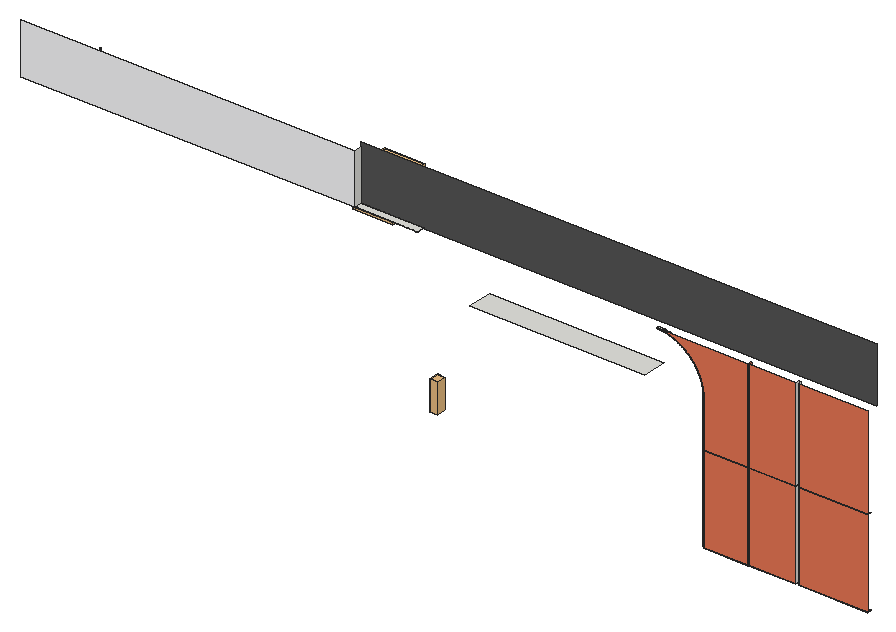
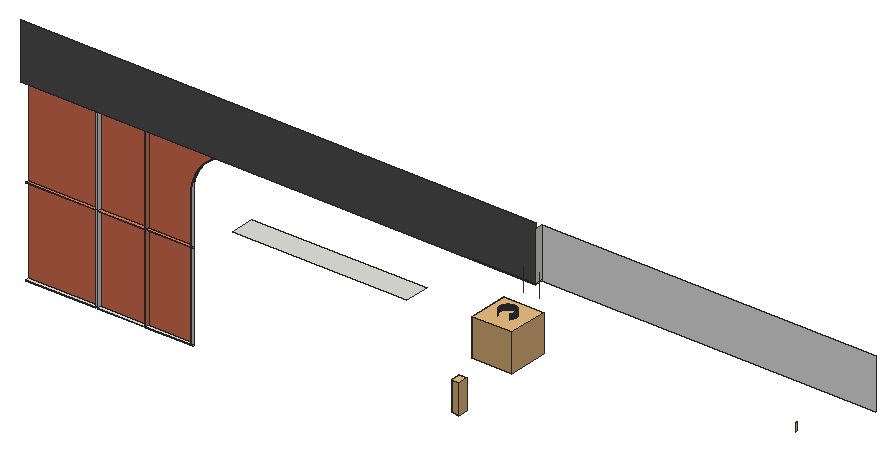
# SketchUp Ruby script. Lengths in inches.
U = 1.inch
M = Sketchup.active_model
def pt(a) = Geom::Point3d.new(a.map { |v| v * U })
def face(e, loops, mat)
  f = e.add_face(loops[0].map { |a| pt(a) })
  loops[1..].each { |l| e.add_face(l.map { |a| pt(a) }).erase! }
  f.material = f.back_material = mat if mat
  f
end
# faces: each face lists its corners as indices into pts; further lists are holes
def faces(e, pts, list, mat = nil) = list.each { |f| face(e, (f[0].is_a?(Array) ? f : [f]).map { |l| l.map { |i| pts[i] } }, mat) }
# xy, xz, yz: faces in a plane at the given z, y or x. An outline is a flat list of corners, or four numbers for a rectangle; further outlines are holes
def ring(l) = l.size == 4 ? [[l[0], l[1]], [l[2], l[1]], [l[2], l[3]], [l[0], l[3]]] : l.each_slice(2).to_a
def flat(e, list, mat, &to3) = list.each { |f| face(e, (f[0].is_a?(Array) ? f : [f]).map { |l| ring(l).map { |u, v| to3.(u, v) } }, mat) }
def xy(e, z, list, mat = nil) = flat(e, list, mat) { |x, y| [x, y, z] }
def xz(e, y, list, mat = nil) = flat(e, list, mat) { |x, z| [x, y, z] }
def yz(e, x, list, mat = nil) = flat(e, list, mat) { |y, z| [x, y, z] }
def lines(e, pts, list) = list.each { |a, b| e.add_line(pt(pts[a]), pt(pts[b])) }
# prism: a flat outline (further loops are holes) pulled along v
def prism(e, loops, v, mat = nil)
  f = face(e, loops, mat); d = Geom::Vector3d.new(v.map { |x| x * U })
  f.pushpull(f.normal.samedirection?(d) ? d.length : -d.length)
end
def box(e, o, s, mat = nil) = prism(e, [[o, [o[0] + s[0], o[1], o[2]], [o[0] + s[0], o[1] + s[1], o[2]], [o[0], o[1] + s[1], o[2]]]], [0, 0, s[2]], mat)
def at(x, y, z, deg = 0) = Geom::Transformation.translation(pt([x, y, z])) * Geom::Transformation.rotation(ORIGIN, Z_AXIS, deg.degrees)
def axes(o, x, y, z) = Geom::Transformation.new([*x, 0, *y, 0, *z, 0, *pt(o).to_a, 1])
def part(name) = M.definitions.add(name)
# library, detail: a bought-in or finely detailed component or shape, given as its bounding box
def library(name, o, s) = part(name).tap { |d| box(d.entities, o, s) }
def detail(e, o, s) = box(e.add_group.entities, o, s)
def put(e, d, t, mat = nil) = e.add_instance(d, t).tap { |i| i.material = mat if mat }
def group(e, t, mat = nil) = e.add_group.tap { |g| g.transformation = t; g.material = mat if mat }.entities
root = M.entities
M.materials.add("1122 AP 7994 PEACH ROSE").color = [254, 227, 201]
M.materials.add("[Cinder Block]").color = [86, 86, 86]
M.materials.add("[Formica Beige]").color = [235, 120, 86]
M.materials.add("[Quartz Light Grey]").color = [251, 251, 252]
c1 = library("9",[-5.85,-5.85,-13.96],[15.28,15.28,13.96])
c2 = library("WALL LIGHT 69",[4.19,4.05,-8.78],[4.61,5.7,17.13])
box(root,[171.19,153,278.82],[23.81,3,0.2])
xy(root,210.57,[[304,152,320.75,152,320.75,153.25,303,153.25,303,153,304,153],[321,152,338.75,153.25],[339.75,152,366,153.25]],"[Formica Beige]")
xy(root,210.82,[[304,152,304,153,303,153,303,153.25,320.75,153.25,320.75,152],[321,152,338.75,153.25],[339.75,152,366,153.25]])
xy(root,243.57,[[304,152,320.75,152,320.75,153.25,303,153.25,303,153,304,153],[321,152,338.75,153.25],[339.75,152,366,153.25]],"[Formica Beige]")
xy(root,243.82,[[304,152,304,153,303,153,303,153.25,320.75,153.25,320.75,152],[321,152,338.75,153.25],[339.75,152,366,153.25]],"[Formica Beige]")
xy(root,260.82,[[215,153,281,162]])
xy(root,278.82,[[286.125,152,286.4,153]])
xz(root,152,[[304,210.82,320.75,243.57],[321,210.82,338.75,243.57],[339.75,210.82,366,243.57],[304,243.82,320.75,243.82,320.75,278.82,286.125,278.82,286.4,278.82,286.68,278.8125,286.96,278.8,287.23,278.78,287.51,278.77,287.79,278.74,288.0625,278.71,288.34,278.68,288.61,278.65,288.89,278.6,289.16,278.56,289.43,278.51,289.71,278.46,290.25,278.34,290.52,278.27,290.78,278.2,291.05,278.13,291.32,278.05,291.58,277.97,291.85,277.88,292.11,277.79,292.37,277.69,292.625,277.6,292.88,277.49,293.14,277.39,293.39,277.27,293.65,277.16,294.15,276.92,294.39,276.79,294.64,276.66,294.88,276.53,295.36,276.25,295.6,276.1,295.83,275.96,296.0625,275.8,296.29,275.65,296.52,275.49,296.74,275.33,297.4,274.82,298.03,274.28,298.24,274.09,298.64,273.71,298.84,273.51,299.03,273.3125,299.22,273.11,299.41,272.91,299.95,272.28,300.12,272.0625,300.29,271.84,300.46,271.62,300.625,271.4,300.79,271.17,300.94,270.94,301.1,270.71,301.24,270.48,301.39,270.24,301.53,270.01,301.67,269.77,301.81,269.52,301.9375,269.28,302.07,269.03,302.1875,268.79,302.31,268.54,302.42,268.28,302.54,268.03,302.64,267.77,302.75,267.52,302.85,267.26,302.94,267,303,266.72,303.13,266.45,303.22,266.16,303.31,265.875,303.39,265.58,303.6,264.71,303.66,264.41,303.72,264.12,303.77,263.82,303.8125,263.52,303.85,263.22,303.89,262.92,303.92,262.625,303.95,262.32,303.97,262.02,304,261.12],[321,243.82,338.75,278.82],
  [339.75,243.82,366,278.82]],"[Formica Beige]")
xz(root,153,[[303,210.57,304,210.82],[303,210.82,304,243.57],[303,243.57,304,243.82],[303,243.82,304,243.82,304,261.12,303.97,262.02,303.95,262.32,303.92,262.625,303.89,262.92,303.85,263.22,303.8125,263.52,303.77,263.82,303.72,264.12,303.66,264.41,303.6,264.71,303.39,265.58,303.31,265.875,303.22,266.16,303.13,266.45,303,266.72]])
xz(root,153,[[45,278.82,171.19,297.82]],"[Quartz Light Grey]")
xz(root,156,[[171.19,278.82,366,299.82]],"[Cinder Block]")
xz(root,174,[[164.84,278.82,164.92,281.82],[164.92,278.82,165,281.82],[165,278.82,165.08,281.82],[165.08,278.82,165.16,281.82]],"1122 AP 7994 PEACH ROSE")
yz(root,55.98,[[176.92,278.82,177,281.82],[177,278.82,177.08,281.82]],"1122 AP 7994 PEACH ROSE")
yz(root,162,[[176.84,278.82,176.92,281.82],[176.92,278.82,177,281.82],[177,278.82,177.08,281.82],[177.08,278.82,177.16,281.82]],"1122 AP 7994 PEACH ROSE")
yz(root,168,[[176.84,278.82,176.92,281.82],[176.92,278.82,177,281.82],[177,278.82,177.08,281.82],[177.08,278.82,177.16,281.82]],"1122 AP 7994 PEACH ROSE")
yz(root,171.19,[[153,278.82,156,297.82]])
yz(root,303,[[153,210.57,153.25,210.82],[153,243.57,153.25,243.82]])
yz(root,304,[[152,210.82,153,243.57],[152,243.82,153,260.82],[152,260.82,153,261.12]])
yz(root,320.75,[[152,210.82,153.25,243.57],[152,243.82,153.25,278.82]],"[Formica Beige]")
yz(root,321,[[152,210.82,153.25,243.57],[152,243.82,153.25,278.82]],"[Formica Beige]")
yz(root,338.75,[[152,210.82,153.25,243.57],[152,243.82,153.25,278.82]])
yz(root,339.75,[[152,210.82,153.25,243.57],[152,243.82,153.25,278.82]])
p = [[303.99,153,261.42],[304,153,261.12],[304,152,261.12],[303.99,152,261.42],[303.98,153,261.72],[303.98,152,261.72],
  [303.97,153,262.02],[303.97,152,262.02],[303.95,153,262.32],[303.95,152,262.32],[303.92,153,262.625],[303.92,152,262.625],
  [303.89,153,262.92],[303.89,152,262.92],[303.85,153,263.22],[303.85,152,263.22],[303.8125,153,263.52],[303.8125,152,263.52],
  [303.77,153,263.82],[303.77,152,263.82],[303.72,153,264.12],[303.72,152,264.12],[303.66,153,264.41],[303.66,152,264.41],
  [303.6,153,264.71],[303.6,152,264.71],[303.53,153,265],[303.53,152,265],[303.46,153,265.29],[303.46,152,265.29],
  [303.39,153,265.58],[303.39,152,265.58],[303.31,153,265.875],[303.31,152,265.875],[303.22,153,266.16],[303.22,152,266.16],
  [303.13,153,266.45],[303.13,152,266.45],[303,153,266.72],[303,152,266.72],[302.94,153,267],[302.94,152,267],
  [302.85,153,267.26],[302.85,152,267.26],[302.75,153,267.52],[302.75,152,267.52],[302.64,153,267.77],[302.64,152,267.77],
  [302.54,153,268.03],[302.54,152,268.03],[302.42,153,268.28],[302.42,152,268.28],[302.31,153,268.54],[302.31,152,268.54],
  [302.1875,153,268.79],[302.1875,152,268.79],[302.07,153,269.03],[302.07,152,269.03],[301.9375,153,269.28],[301.9375,152,269.28],
  [301.81,153,269.52],[301.81,152,269.52],[301.67,153,269.77],[301.67,152,269.77],[301.53,153,270.01],[301.53,152,270.01],
  [301.39,153,270.24],[301.39,152,270.24],[301.24,153,270.48],[301.24,152,270.48],[301.1,153,270.71],[301.1,152,270.71],
  [300.94,153,270.94],[300.94,152,270.94],[300.79,153,271.17],[300.79,152,271.17],[300.625,153,271.4],[300.625,152,271.4],
  [300.46,153,271.62],[300.46,152,271.62],[300.29,153,271.84],[300.29,152,271.84],[300.12,153,272.0625],[300.12,152,272.0625],
  [299.95,153,272.28],[299.95,152,272.28],[299.77,153,272.49],[299.77,152,272.49],[299.59,153,272.7],[299.59,152,272.7],
  [299.41,153,272.91],[299.41,152,272.91],[299.22,153,273.11],[299.22,152,273.11],[299.03,153,273.3125],[299.03,152,273.3125],
  [298.84,153,273.51],[298.84,152,273.51],[298.64,153,273.71],[298.64,152,273.71],[298.44,153,273.9],[298.44,152,273.9],
  [298.24,153,274.09],[298.24,152,274.09],[298.03,153,274.28],[298.03,152,274.28],[297.82,153,274.46],[297.82,152,274.46],
  [297.61,153,274.64],[297.61,152,274.64],[297.4,153,274.82],[297.4,152,274.82],[297.18,153,274.99],[297.18,152,274.99],
  [296.96,153,275.16],[296.96,152,275.16],[296.74,153,275.33],[296.74,152,275.33],[296.52,153,275.49],[296.52,152,275.49],
  [296.29,153,275.65],[296.29,152,275.65],[296.0625,153,275.8],[296.0625,152,275.8],[295.83,153,275.96],[295.83,152,275.96],
  [295.6,153,276.1],[295.6,152,276.1],[295.36,153,276.25],[295.36,152,276.25],[295.12,153,276.39],[295.12,152,276.39],
  [294.88,153,276.53],[294.88,152,276.53],[294.64,153,276.66],[294.64,152,276.66],[294.39,153,276.79],[294.39,152,276.79],
  [294.15,153,276.92],[294.15,152,276.92],[293.9,153,277.04],[293.9,152,277.04],[293.65,153,277.16],[293.65,152,277.16],
  [293.39,153,277.27],[293.39,152,277.27],[293.14,153,277.39],[293.14,152,277.39],[292.88,153,277.49],[292.88,152,277.49],
  [292.625,153,277.6],[292.625,152,277.6],[292.37,153,277.69],[292.37,152,277.69],[292.11,153,277.79],[292.11,152,277.79],
  [291.85,153,277.88],[291.85,152,277.88],[291.58,153,277.97],[291.58,152,277.97],[291.05,153,278.13],[291.32,153,278.05],
  [291.32,152,278.05],[291.05,152,278.13],[290.78,153,278.2],[290.78,152,278.2],[290.52,153,278.27],[290.52,152,278.27],
  [289.98,153,278.4],[290.25,153,278.34],[290.25,152,278.34],[289.98,152,278.4],[289.71,153,278.46],[289.71,152,278.46],
  [289.16,153,278.56],[289.43,153,278.51],[289.43,152,278.51],[289.16,152,278.56],[288.34,153,278.68],[288.61,153,278.65],
  [288.61,152,278.65],[288.34,152,278.68],[288.89,153,278.6],[288.89,152,278.6],[287.51,153,278.77],[287.79,153,278.74],
  [287.79,152,278.74],[287.51,152,278.77],[288.0625,153,278.71],[288.0625,152,278.71],[286.4,153,278.82],[286.68,153,278.8125],
  [286.68,152,278.8125],[286.4,152,278.82],[286.96,153,278.8],[286.96,152,278.8],[287.23,153,278.78],[287.23,152,278.78],
  [164.53,174.04,278.82],[164.45,174.05,278.82],[164.45,174.05,281.82],[164.53,174.04,281.82],[164.61,174.03,278.82],[164.61,174.03,281.82],
  [164.6875,174.02,278.82],[164.6875,174.02,281.82],[164.76,174.01,278.82],[164.76,174.01,281.82],[164.84,174,278.82],[164.84,174,281.82],
  [165.24,174.01,278.82],[165.16,174,278.82],[165.16,174,281.82],[165.24,174.01,281.82],[165.3125,174.02,278.82],[165.3125,174.02,281.82],
  [165.39,174.03,278.82],[165.39,174.03,281.82],[165.47,174.04,278.82],[165.47,174.04,281.82],[165.55,174.05,278.82],[165.55,174.05,281.82],
  [164.07,174.15,278.82],[164,174.17,278.82],[164,174.17,281.82],[164.07,174.15,281.82],[164.15,174.125,278.82],[164.15,174.125,281.82],
  [164.22,174.1,278.82],[164.22,174.1,281.82],[164.3,174.08,278.82],[164.3,174.08,281.82],[164.375,174.07,278.82],[164.375,174.07,281.82],
  [165.625,174.07,278.82],[165.625,174.07,281.82],[165.7,174.08,278.82],[165.7,174.08,281.82],[165.78,174.1,278.82],[165.78,174.1,281.82],
  [165.85,174.125,278.82],[165.85,174.125,281.82],[165.93,174.15,278.82],[165.93,174.15,281.82],[166,174.17,278.82],[166,174.17,281.82],
  [163.85,174.23,278.82],[163.78,174.26,278.82],[163.78,174.26,281.82],[163.85,174.23,281.82],[163.92,174.2,278.82],[163.92,174.2,281.82],
  [166.08,174.2,278.82],[166.08,174.2,281.82],[166.15,174.23,278.82],[166.15,174.23,281.82],[166.22,174.26,278.82],[166.22,174.26,281.82],
  [163.64,174.33,278.82],[163.57,174.36,278.82],[163.57,174.36,281.82],[163.64,174.33,281.82],[163.71,174.29,278.82],[163.71,174.29,281.82],
  [166.29,174.29,278.82],[166.29,174.29,281.82],[166.36,174.33,278.82],[166.36,174.33,281.82],[166.43,174.36,278.82],[166.43,174.36,281.82],
  [163.43,174.44,278.82],[163.37,174.48,278.82],[163.37,174.48,281.82],[163.43,174.44,281.82],[163.5,174.4,278.82],[163.5,174.4,281.82],
  [166.5,174.4,278.82],[166.5,174.4,281.82],[166.57,174.44,278.82],[166.57,174.44,281.82],[166.63,174.48,278.82],[166.63,174.48,281.82],
  [163.3,174.53,278.82],[163.24,174.57,278.82],[163.24,174.57,281.82],[163.3,174.53,281.82],[166.7,174.53,278.82],[166.7,174.53,281.82],
  [166.76,174.57,278.82],[166.76,174.57,281.82],[163.17,174.62,278.82],[163.11,174.67,278.82],[163.11,174.67,281.82],[163.17,174.62,281.82],
  [166.83,174.62,278.82],[166.83,174.62,281.82],[166.89,174.67,278.82],[166.89,174.67,281.82],[163.05,174.72,278.82],[162.99,174.77,278.82],
  [162.99,174.77,281.82],[163.05,174.72,281.82],[166.95,174.72,278.82],[166.95,174.72,281.82],[167.01,174.77,278.82],[167.01,174.77,281.82],
  [162.93,174.82,278.82],[162.88,174.88,278.82],[162.88,174.88,281.82],[162.93,174.82,281.82],[167.07,174.82,278.82],[167.07,174.82,281.82],
  [167.12,174.88,278.82],[167.12,174.88,281.82],[162.82,174.93,278.82],[162.77,174.99,278.82],[162.77,174.99,281.82],[162.82,174.93,281.82],
  [167.18,174.93,278.82],[167.18,174.93,281.82],[167.23,174.99,278.82],[167.23,174.99,281.82],[162.72,175.05,278.82],[162.72,175.05,281.82],
  [167.28,175.05,278.82],[167.28,175.05,281.82],[162.67,175.11,278.82],[162.62,175.17,278.82],[162.62,175.17,281.82],[162.67,175.11,281.82],
  [167.33,175.11,278.82],[167.33,175.11,281.82],[167.38,175.17,278.82],[167.38,175.17,281.82],[162.57,175.24,278.82],[162.53,175.3,278.82],
  [162.53,175.3,281.82],[162.57,175.24,281.82],[167.43,175.24,278.82],[167.43,175.24,281.82],[167.47,175.3,278.82],[167.47,175.3,281.82],
  [162.48,175.37,278.82],[162.48,175.37,281.82],[167.52,175.37,278.82],[167.52,175.37,281.82],[162.44,175.43,278.82],[162.4,175.5,278.82],
  [162.4,175.5,281.82],[162.44,175.43,281.82],[167.56,175.43,278.82],[167.56,175.43,281.82],[167.6,175.5,278.82],[167.6,175.5,281.82],
  [162.36,175.57,278.82],[162.36,175.57,281.82],[167.64,175.57,278.82],[167.64,175.57,281.82],[162.33,175.64,278.82],[162.29,175.71,278.82],
  [162.29,175.71,281.82],[162.33,175.64,281.82],[167.67,175.64,278.82],[167.67,175.64,281.82],[167.71,175.71,278.82],[167.71,175.71,281.82],
  [162.26,175.78,278.82],[162.26,175.78,281.82],[167.74,175.78,278.82],[167.74,175.78,281.82],[162.23,175.85,278.82],[162.23,175.85,281.82],
  [167.77,175.85,278.82],[167.77,175.85,281.82],[162.2,175.92,278.82],[162.17,176,278.82],[162.17,176,281.82],[162.2,175.92,281.82],
  [167.8,175.92,278.82],[167.8,175.92,281.82],[167.83,176,278.82],[167.83,176,281.82],[162.15,176.07,278.82],[162.15,176.07,281.82],
  [167.85,176.07,278.82],[167.85,176.07,281.82],[162.125,176.15,278.82],[162.1,176.22,278.82],[162.1,176.22,281.82],[162.125,176.15,281.82],
  [167.875,176.15,278.82],[167.875,176.15,281.82],[167.9,176.22,278.82],[167.9,176.22,281.82],[162.08,176.3,278.82],[162.08,176.3,281.82],
  [167.92,176.3,278.82],[167.92,176.3,281.82],[162.07,176.375,278.82],[162.07,176.375,281.82],[167.93,176.375,278.82],[167.93,176.375,281.82],
  [162.05,176.45,278.82],[162.05,176.45,281.82],[167.95,176.45,278.82],[167.95,176.45,281.82],[162.04,176.53,278.82],[162.03,176.61,278.82],
  [162.03,176.61,281.82],[162.04,176.53,281.82],[167.96,176.53,278.82],[167.96,176.53,281.82],[167.97,176.61,278.82],[167.97,176.61,281.82],
  [162.02,176.6875,278.82],[162.02,176.6875,281.82],[167.98,176.6875,278.82],[167.98,176.6875,281.82],[162.01,176.76,278.82],[162.01,176.76,281.82],
  [167.99,176.76,278.82],[167.99,176.76,281.82],[162,176.84,278.82],[162,176.84,281.82],[168,176.84,278.82],[168,176.84,281.82],
  [162,177.16,278.82],[162.01,177.24,278.82],[162.01,177.24,281.82],[162,177.16,281.82],[162.02,177.3125,278.82],[162.02,177.3125,281.82],
  [167.98,177.3125,278.82],[167.99,177.24,278.82],[167.99,177.24,281.82],[167.98,177.3125,281.82],[168,177.16,278.82],[168,177.16,281.82],
  [162.03,177.39,278.82],[162.03,177.39,281.82],[167.97,177.39,278.82],[167.97,177.39,281.82],[162.04,177.47,278.82],[162.04,177.47,281.82],
  [167.96,177.47,278.82],[167.96,177.47,281.82],[162.05,177.55,278.82],[162.05,177.55,281.82],[162.07,177.625,278.82],[162.07,177.625,281.82],
  [167.93,177.625,278.82],[167.95,177.55,278.82],[167.95,177.55,281.82],[167.93,177.625,281.82],[162.08,177.7,278.82],[162.08,177.7,281.82],
  [167.92,177.7,278.82],[167.92,177.7,281.82],[162.1,177.78,278.82],[162.1,177.78,281.82],[167.9,177.78,278.82],[167.9,177.78,281.82],
  [162.125,177.85,278.82],[162.125,177.85,281.82],[167.875,177.85,278.82],[167.875,177.85,281.82],[162.15,177.93,278.82],[162.15,177.93,281.82],
  [162.17,178,278.82],[162.17,178,281.82],[167.83,178,278.82],[167.85,177.93,278.82],[167.85,177.93,281.82],[167.83,178,281.82],
  [162.2,178.08,278.82],[162.2,178.08,281.82],[167.8,178.08,278.82],[167.8,178.08,281.82],[162.23,178.15,278.82],[162.23,178.15,281.82],
  [162.26,178.22,278.82],[162.26,178.22,281.82],[167.74,178.22,278.82],[167.77,178.15,278.82],[167.77,178.15,281.82],[167.74,178.22,281.82],
  [162.29,178.29,278.82],[162.29,178.29,281.82],[167.71,178.29,278.82],[167.71,178.29,281.82],[162.33,178.36,278.82],[162.33,178.36,281.82],
  [167.67,178.36,278.82],[167.67,178.36,281.82],[162.36,178.43,278.82],[162.36,178.43,281.82],[162.4,178.5,278.82],[162.4,178.5,281.82],
  [167.6,178.5,278.82],[167.64,178.43,278.82],[167.64,178.43,281.82],[167.6,178.5,281.82],[162.44,178.57,278.82],[162.44,178.57,281.82],
  [167.56,178.57,278.82],[167.56,178.57,281.82],[162.48,178.63,278.82],[162.48,178.63,281.82],[162.53,178.7,278.82],[162.53,178.7,281.82],
  [167.47,178.7,278.82],[167.52,178.63,278.82],[167.52,178.63,281.82],[167.47,178.7,281.82],[162.57,178.76,278.82],[162.57,178.76,281.82],
  [167.43,178.76,278.82],[167.43,178.76,281.82],[162.62,178.83,278.82],[162.62,178.83,281.82],[162.67,178.89,278.82],[162.67,178.89,281.82],
  [167.33,178.89,278.82],[167.38,178.83,278.82],[167.38,178.83,281.82],[167.33,178.89,281.82],[162.72,178.95,278.82],[162.72,178.95,281.82],
  [162.77,179.01,278.82],[162.77,179.01,281.82],[167.23,179.01,278.82],[167.28,178.95,278.82],[167.28,178.95,281.82],[167.23,179.01,281.82],
  [171,162,278.82],[171,162,287.82],[165,162,278.82],[165,162,287.82],[171.19,153,278.82],[195,153,278.82],
  [195,156,278.82]]
faces(root,p,[[0,1,2,3],[4,0,3,5],[6,4,5,7],[8,6,7,9],[10,8,9,11],[12,10,11,13],[14,12,13,15],[16,14,15,17],
  [18,16,17,19],[20,18,19,21],[22,20,21,23],[24,22,23,25],[26,24,25,27],[28,26,27,29],[30,28,29,31],[32,30,31,33],
  [34,32,33,35],[36,34,35,37],[38,36,37,39],[40,38,39,41],[42,40,41,43],[44,42,43,45],[46,44,45,47],[48,46,47,49],
  [50,48,49,51],[52,50,51,53],[54,52,53,55],[56,54,55,57],[58,56,57,59],[60,58,59,61],[62,60,61,63],[64,62,63,65],
  [66,64,65,67],[68,66,67,69],[70,68,69,71],[72,70,71,73],[74,72,73,75],[76,74,75,77],[78,76,77,79],[80,78,79,81],
  [82,80,81,83],[84,82,83,85],[86,84,85,87],[88,86,87,89],[90,88,89,91],[92,90,91,93],[94,92,93,95],[96,94,95,97],
  [98,96,97,99],[100,98,99,101],[102,100,101,103],[104,102,103,105],[106,104,105,107],[108,106,107,109],[110,108,109,111],[112,110,111,113],
  [114,112,113,115],[116,114,115,117],[118,116,117,119],[120,118,119,121],[122,120,121,123],[124,122,123,125],[126,124,125,127],[128,126,127,129],
  [130,128,129,131],[132,130,131,133],[134,132,133,135],[136,134,135,137],[138,136,137,139],[140,138,139,141],[142,140,141,143],[144,142,143,145],
  [146,144,145,147],[148,146,147,149],[150,148,149,151],[152,150,151,153],[154,152,153,155],[156,154,155,157],[158,156,157,159],[160,161,162,163],
  [161,158,159,162],[164,160,163,165],[166,164,165,167],[168,169,170,171],[169,166,167,170],[172,168,171,173],[174,175,176,177],[175,172,173,176],
  [178,179,180,181],[179,182,183,180],[182,174,177,183],[184,185,186,187],[185,188,189,186],[188,178,181,189],[190,191,192,193],[191,194,195,192],
  [194,196,197,195],[196,184,187,197]])
faces(root,p,[[198,199,200,201],[202,198,201,203],[204,202,203,205],[206,204,205,207],[208,206,207,209],[210,211,212,213],[214,210,213,215],[216,214,215,217],
  [218,216,217,219],[220,218,219,221],[222,223,224,225],[226,222,225,227],[228,226,227,229],[230,228,229,231],[232,230,231,233],[199,232,233,200],
  [234,220,221,235],[236,234,235,237],[238,236,237,239],[240,238,239,241],[242,240,241,243],[244,242,243,245],[246,247,248,249],[250,246,249,251],
  [223,250,251,224],[252,244,245,253],[254,252,253,255],[256,254,255,257],[258,259,260,261],[262,258,261,263],[247,262,263,248],[264,256,257,265],
  [266,264,265,267],[268,266,267,269],[270,271,272,273],[274,270,273,275],[259,274,275,260],[276,268,269,277],[278,276,277,279],[280,278,279,281],
  [282,283,284,285],[271,282,285,272],[286,280,281,287],[288,286,287,289],[290,291,292,293],[283,290,293,284],[294,288,289,295],[296,294,295,297],
  [298,299,300,301],[291,298,301,292],[302,296,297,303],[304,302,303,305],[306,307,308,309],[299,306,309,300],[310,304,305,311],[312,310,311,313],
  [314,315,316,317],[307,314,317,308],[318,312,313,319],[320,318,319,321],[315,322,323,316],[324,320,321,325],[326,327,328,329],[322,326,329,323],
  [330,324,325,331],[332,330,331,333],[334,335,336,337],[327,334,337,328],[338,332,333,339],[340,338,339,341],[335,342,343,336],[344,340,341,345],
  [346,347,348,349],[342,346,349,343],[350,344,345,351],[352,350,351,353],[347,354,355,348],[356,352,353,357],[358,359,360,361],[354,358,361,355],
  [362,356,357,363],[364,362,363,365],[359,366,367,360],[368,364,365,369],[366,370,371,367],[372,368,369,373],[374,375,376,377],[370,374,377,371],
  [378,372,373,379],[380,378,379,381],[375,382,383,376],[384,380,381,385],[386,387,388,389],[382,386,389,383],[390,384,385,391],[392,390,391,393],
  [387,394,395,388],[396,392,393,397],[394,398,399,395],[400,396,397,401],[398,402,403,399],[404,400,401,405],[406,407,408,409],[402,406,409,403],
  [410,404,405,411],[412,410,411,413],[407,414,415,408],[416,412,413,417],[414,418,419,415],[420,416,417,421],[418,422,423,419],[424,420,421,425],
  [426,427,428,429],[427,430,431,428],[432,433,434,435],[433,436,437,434],[430,438,439,431],[440,432,435,441],[438,442,443,439],[444,440,441,445],
  [442,446,447,443],[446,448,449,447],[450,451,452,453],[451,444,445,452],[448,454,455,449],[456,450,453,457],[454,458,459,455],[460,456,457,461],
  [458,462,463,459],[464,460,461,465],[462,466,467,463],[466,468,469,467],[470,471,472,473],[471,464,465,472],[468,474,475,469],[476,470,473,477],
  [474,478,479,475],[478,480,481,479],[482,483,484,485],[483,476,477,484],[480,486,487,481],[488,482,485,489],[486,490,491,487],[492,488,489,493],
  [490,494,495,491],[494,496,497,495],[498,499,500,501],[499,492,493,500],[496,502,503,497],[504,498,501,505],[502,506,507,503],[506,508,509,507],
  [510,511,512,513],[511,504,505,512],[508,514,515,509],[516,510,513,517],[514,518,519,515],[518,520,521,519],[522,523,524,525],[523,516,517,524],
  [520,526,527,521],[526,528,529,527],[530,531,532,533],[531,522,525,532]],"1122 AP 7994 PEACH ROSE")
lines(root,p,[[534,535],[536,537],[538,539],[539,540]])
put(root,c1,at(163.21,175.21,280.07))
put(root,c2,axes([199.84,146.66,227.9],[0.65,0,0],[0,0.65,0],[0,0,0.65]))
